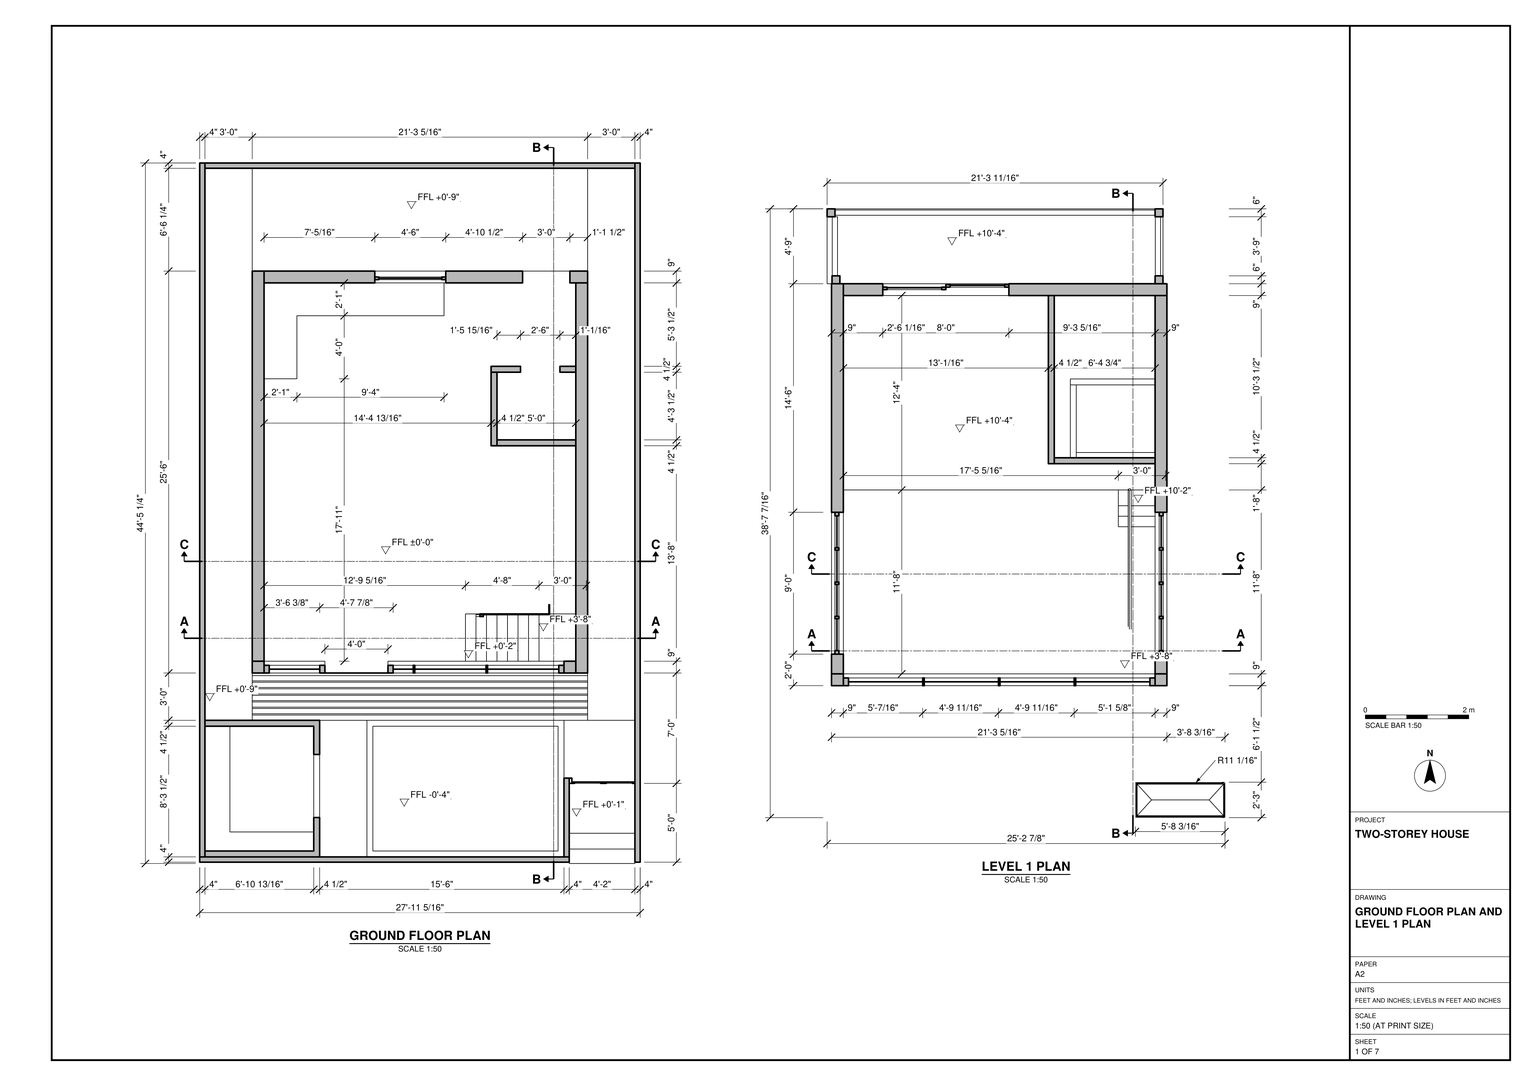
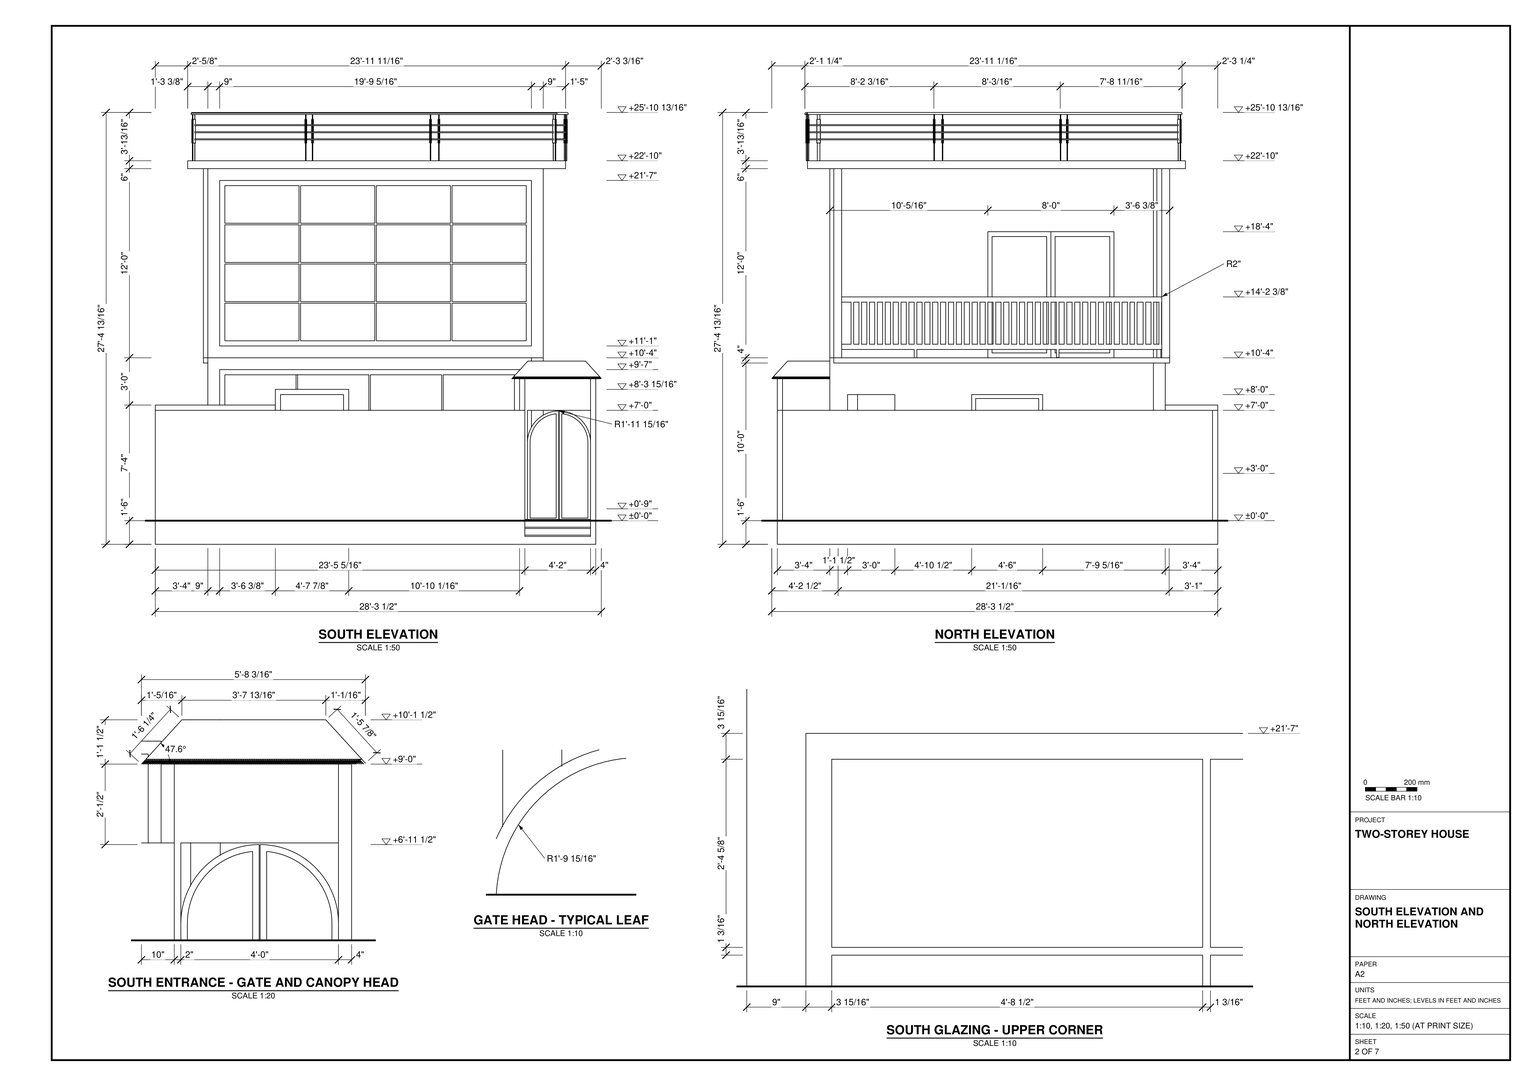
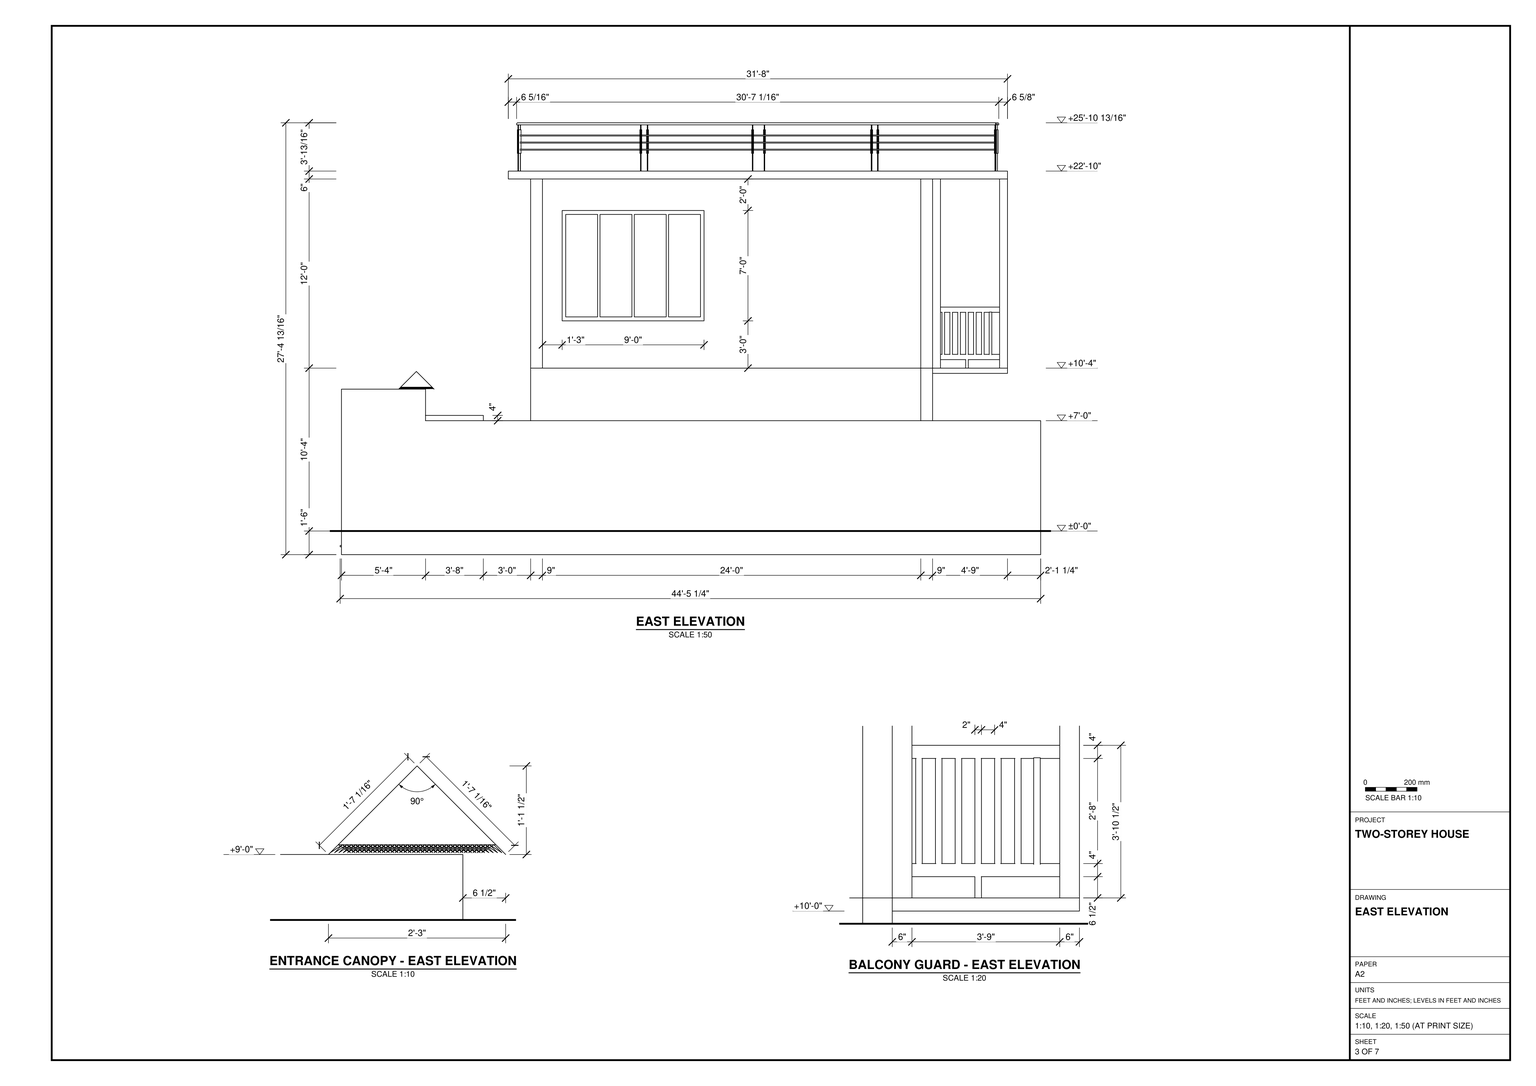
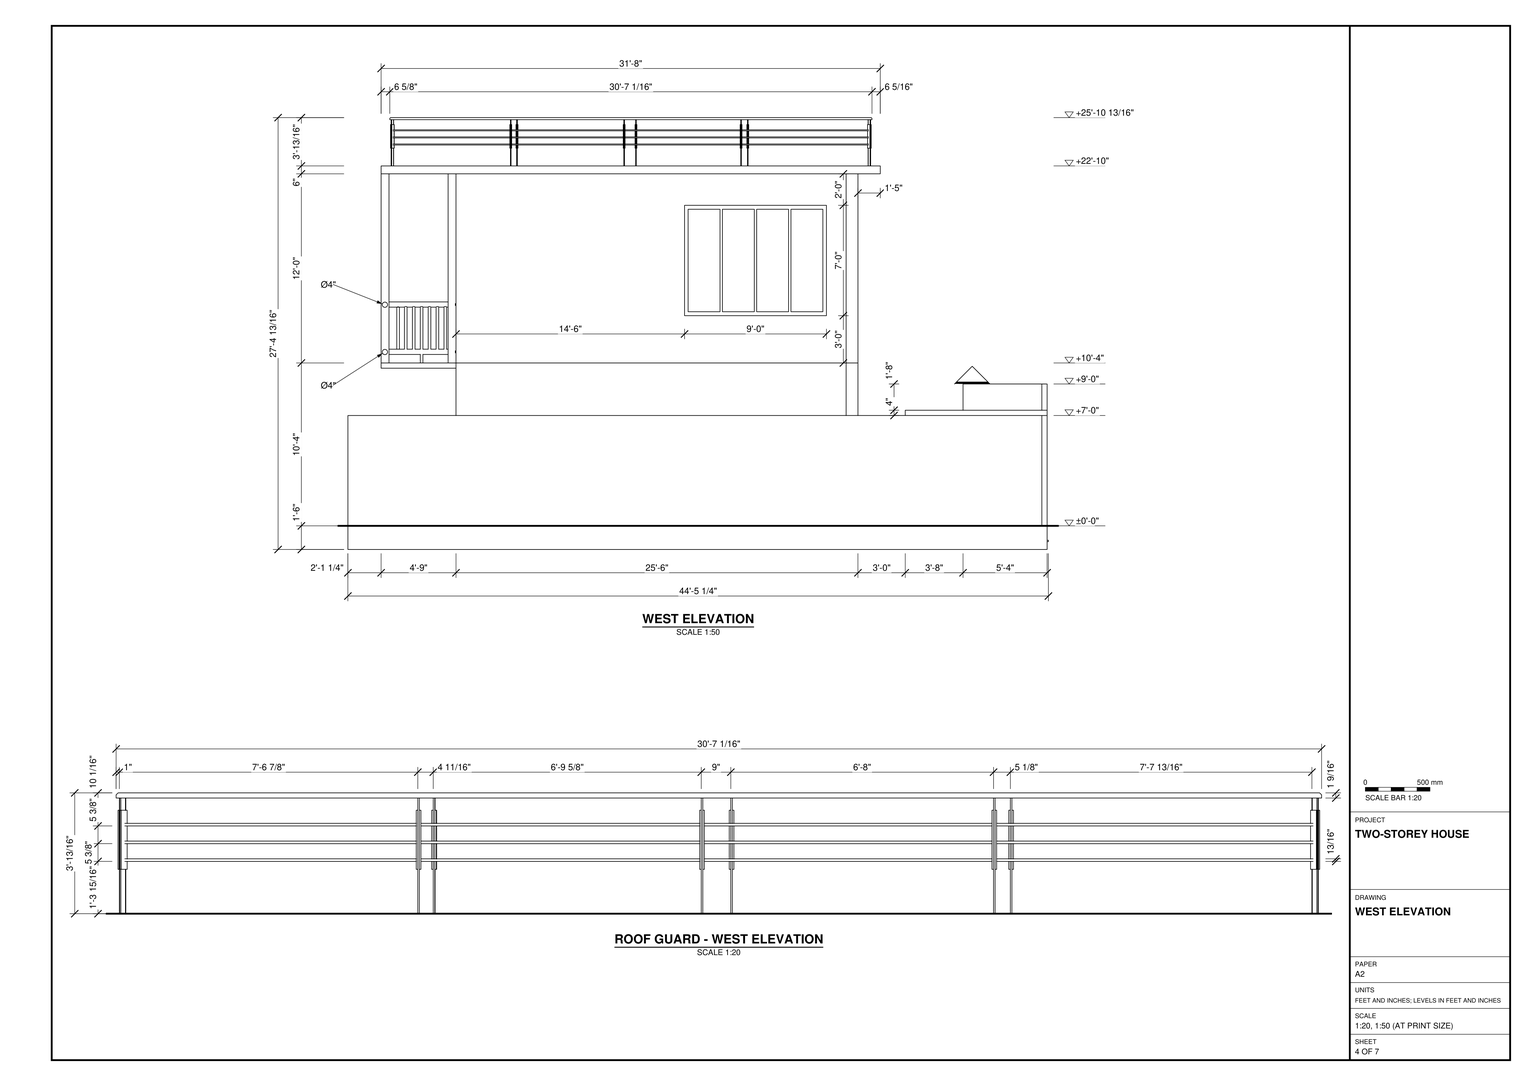
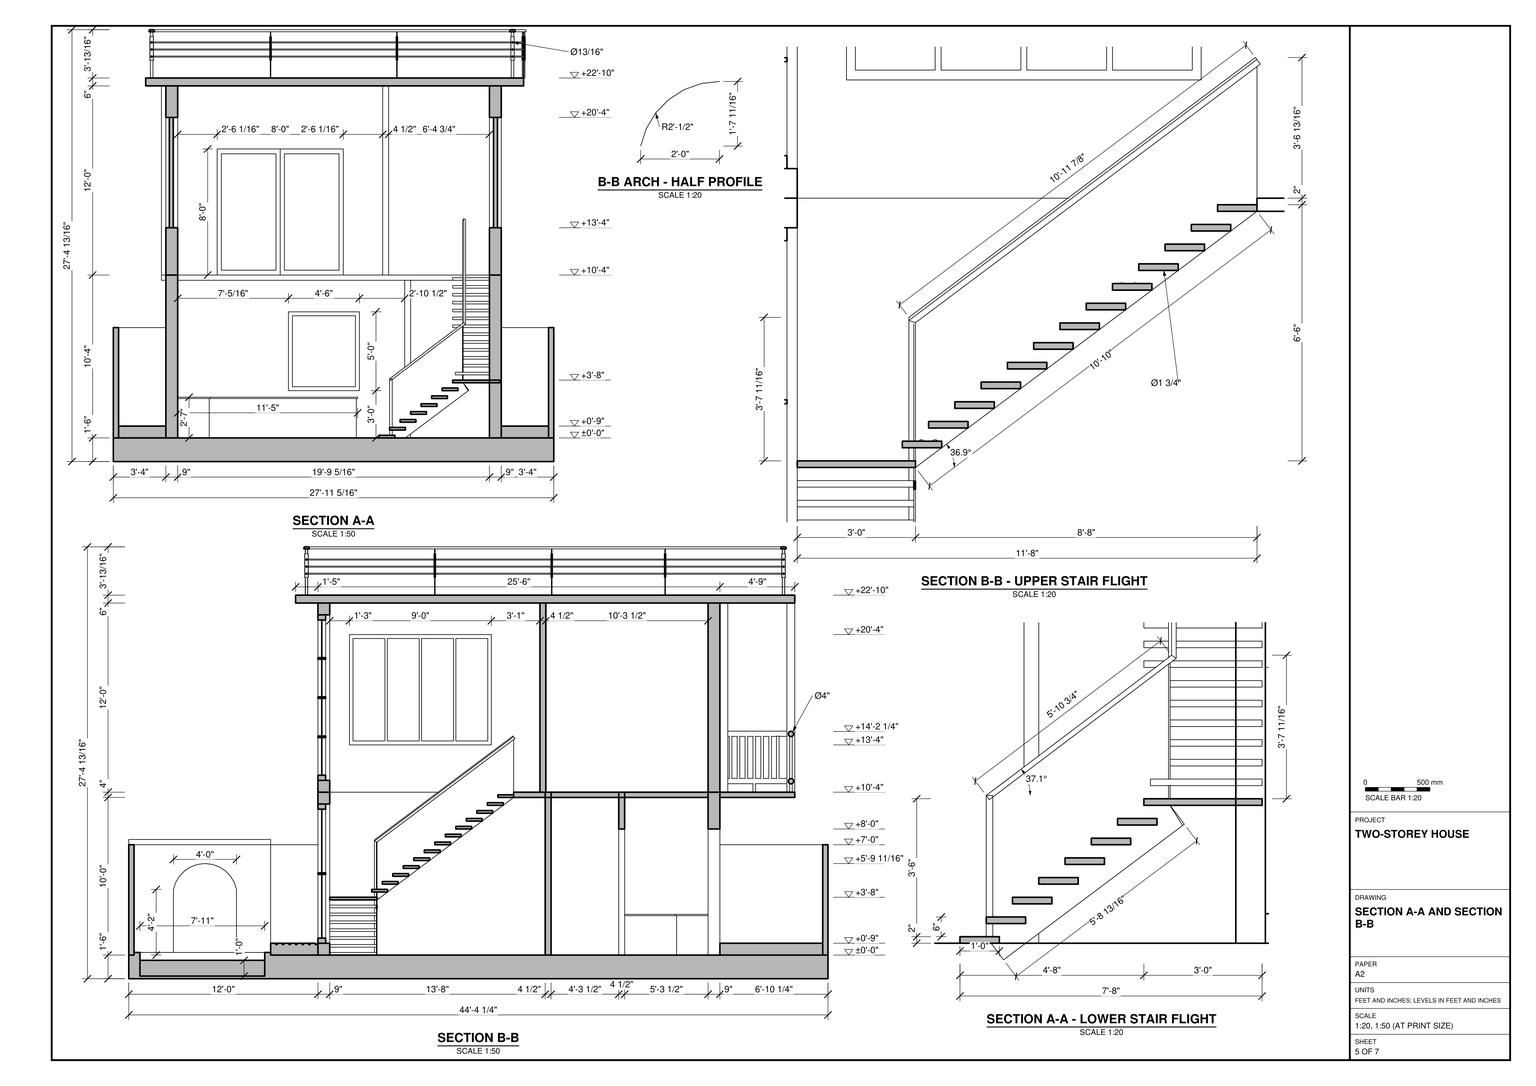
Build the house and its walled court in SketchUp using task_files/diagram_01.pdf. Work in feet and inches. Orient the model with the south frontage along the x-axis and the site depth along the y-axis. The complete model, including the site base and roof guard, is 28'-3 1/2" wide, 44'-5 1/4" deep and 27'-4 13/16" high. Set the ground floor at ±0'-0" and the upper floor at +10'-4".

Lay out the site walls, rectangular pool, adjacent enclosure and stepped approach between the south gate and the house. Give the gate its paired arched leaves and small pitched canopy. Build the floor slabs, exterior walls and interior partitions to the thicknesses drawn. Fit the stair and landings along the east side, leaving the south part of the interior open to the floor below. Match the door and window openings to the plans and elevations, including the grid of glazing on the upper south face. Model the projecting north balcony with its vertical guard members and the flat roof with its horizontal rails. Include built-in joinery and main furniture where shown, following their drawn footprints. Decor and loose items may be any suitable library components.

Keep shell elements and individual furniture or joinery pieces in separate groups or components, and use components for repeated parts. Save one SketchUp model as output_files/two_storey_house_with_a_gated_pool_court.skp.

# SketchUp Ruby script. Lengths in inches.
U = 1.inch
M = Sketchup.active_model
def pt(a) = Geom::Point3d.new(a.map { |v| v * U })
def face(e, loops, mat)
  f = e.add_face(loops[0].map { |a| pt(a) })
  loops[1..].each { |l| e.add_face(l.map { |a| pt(a) }).erase! }
  f.material = f.back_material = mat if mat
  f
end
# faces: each face lists its corners as indices into pts; further lists are holes
def faces(e, pts, list, mat = nil) = list.each { |f| face(e, (f[0].is_a?(Array) ? f : [f]).map { |l| l.map { |i| pts[i] } }, mat) }
# xy, xz, yz: faces in a plane at the given z, y or x. An outline is a flat list of corners, or four numbers for a rectangle; further outlines are holes
def ring(l) = l.size == 4 ? [[l[0], l[1]], [l[2], l[1]], [l[2], l[3]], [l[0], l[3]]] : l.each_slice(2).to_a
def flat(e, list, mat, &to3) = list.each { |f| face(e, (f[0].is_a?(Array) ? f : [f]).map { |l| ring(l).map { |u, v| to3.(u, v) } }, mat) }
def xy(e, z, list, mat = nil) = flat(e, list, mat) { |x, y| [x, y, z] }
def xz(e, y, list, mat = nil) = flat(e, list, mat) { |x, z| [x, y, z] }
def yz(e, x, list, mat = nil) = flat(e, list, mat) { |y, z| [x, y, z] }
def lines(e, pts, list) = list.each { |a, b| e.add_line(pt(pts[a]), pt(pts[b])) }
# prism: a flat outline (further loops are holes) pulled along v
def prism(e, loops, v, mat = nil)
  f = face(e, loops, mat); d = Geom::Vector3d.new(v.map { |x| x * U })
  f.pushpull(f.normal.samedirection?(d) ? d.length : -d.length)
end
def box(e, o, s, mat = nil) = prism(e, [[o, [o[0] + s[0], o[1], o[2]], [o[0] + s[0], o[1] + s[1], o[2]], [o[0], o[1] + s[1], o[2]]]], [0, 0, s[2]], mat)
def at(x, y, z, deg = 0) = Geom::Transformation.translation(pt([x, y, z])) * Geom::Transformation.rotation(ORIGIN, Z_AXIS, deg.degrees)
def axes(o, x, y, z) = Geom::Transformation.new([*x, 0, *y, 0, *z, 0, *pt(o).to_a, 1])
def part(name) = M.definitions.add(name)
# library, detail: a bought-in or finely detailed component or shape, given as its bounding box
def library(name, o, s) = part(name).tap { |d| box(d.entities, o, s) }
def detail(e, o, s) = box(e.add_group.entities, o, s)
def put(e, d, t, mat = nil) = e.add_instance(d, t).tap { |i| i.material = mat if mat }
def group(e, t, mat = nil) = e.add_group.tap { |g| g.transformation = t; g.material = mat if mat }.entities
root = M.entities
M.materials.add("  cane").color = [150, 130, 69]
M.materials.add("[Aluminum]").color = [179, 179, 179]
M.materials.add("[Color A01]").color = [255, 204, 204]
M.materials.add("[Color A08]").color = [102, 0, 0]
M.materials.add("[Color C07]").color = [153, 76, 0]
M.materials.add("[Color F02]").color = [204, 255, 153]
M.materials.add("[Color M02]").color = [198, 198, 198]
M.materials.add("[Color M04]").color = [142, 142, 142]
M.materials.add("[Color M06]").color = [86, 86, 86]
M.materials.add("[Color M07]").color = [58, 58, 58]
M.materials.add("[Color M08]").color = [30, 30, 30]
M.materials.add("[Translucent Glass Gray]").color = [128, 128, 128]
M.materials["[Translucent Glass Gray]"].alpha = 0.1
M.materials.add("[Translucent Glass Gray]1").color = [128, 128, 128]
M.materials["[Translucent Glass Gray]1"].alpha = 0.5
M.materials.add("[Water Pool]").color = [64, 149, 167]
M.materials.add("[Wood Veneer 01]").color = [120, 70, 37]
M.materials.add("[Wood Veneer 02]").color = [190, 128, 91]
c1 = part("Group60\#2")
xy(c1.entities,0,[[-110.22,-49.0625,-71.78,-0.59],[-15.9,-49.0625,-0.59,-0.59],[0.59,-49.0625,54.8125,-0.59],[56,-49.0625,110.22,-0.59],[-110.22,-0.59,-71.78,0.59],
  [-110.22,0.59,-110.22,49.0625,-56,49.0625,-56,37.9375,-71.78,37.9375,-71.78,0.59],[-15.9,0.59,-15.9,37.9375,-54.8125,37.9375,-54.8125,49.0625,-0.59,49.0625,-0.59,0.59],[0.59,0.59,54.8125,49.0625],[56,0.59,110.22,49.0625],[-56,37.9375,-54.8125,49.0625]])
c2 = part("Group59\#1")
xy(c2.entities,0,[[[-114.16,-53,-114.16,53,114.16,53,114.16,-53,-19.84,-53,-19.84,34,-67.84,34,-67.84,-53],[-110.22,-49.0625,-71.78,-49.0625,-71.78,37.9375,-15.9,37.9375,-15.9,0.59,-0.59,0.59,-0.59,49.0625,-110.22,49.0625],[56,-49.0625,110.22,-0.59],[0.59,-49.0625,54.8125,-0.59],[56,0.59,110.22,49.0625],[0.59,0.59,54.8125,49.0625],[-15.9,-49.0625,-0.59,-0.59]]])
xy(c2.entities,5.875,[[[-114.16,-53,-67.84,-53,-67.84,34,-19.84,34,-19.84,-53,114.16,-53,114.16,53,-114.16,53],[-110.22,-49.0625,-110.22,49.0625,-0.59,49.0625,-0.59,0.59,-15.9,0.59,-15.9,37.9375,-71.78,37.9375,-71.78,-49.0625],[56,-49.0625,110.22,-0.59],[0.59,-49.0625,54.8125,-0.59],[56,0.59,110.22,49.0625],[0.59,0.59,54.8125,49.0625],[-15.9,-49.0625,-0.59,-0.59]]])
xz(c2.entities,-53,[[-114.16,0,-67.84,5.875],[-19.84,0,114.16,5.875]])
xz(c2.entities,-49.0625,[[-110.22,0,-71.78,5.875],[-15.9,0,-0.59,5.875],[0.59,0,54.8125,5.875],[56,0,110.22,5.875]])
xz(c2.entities,-0.59,[[-15.9,0,-0.59,5.875],[0.59,0,54.8125,5.875],[56,0,110.22,5.875]])
xz(c2.entities,0.59,[[-15.9,0,-0.59,5.875],[0.59,0,54.8125,5.875],[56,0,110.22,5.875]])
xz(c2.entities,34,[[-67.84,0,-19.84,5.875]])
xz(c2.entities,37.9375,[[-71.78,0,-15.9,5.875]])
xz(c2.entities,49.0625,[[-110.22,0,-0.59,5.875],[0.59,0,54.8125,5.875],[56,0,110.22,5.875]])
xz(c2.entities,53,[[-114.16,0,114.16,5.875]])
yz(c2.entities,-114.16,[[-53,0,53,5.875]])
yz(c2.entities,-110.22,[[-49.0625,0,49.0625,5.875]])
yz(c2.entities,-71.78,[[-49.0625,0,37.9375,5.875]])
yz(c2.entities,-67.84,[[-53,0,34,5.875]])
yz(c2.entities,-19.84,[[-53,0,34,5.875]])
yz(c2.entities,-15.9,[[-49.0625,0,-0.59,5.875],[0.59,0,37.9375,5.875]])
yz(c2.entities,-0.59,[[-49.0625,0,-0.59,5.875],[0.59,0,49.0625,5.875]])
yz(c2.entities,0.59,[[-49.0625,0,-0.59,5.875],[0.59,0,49.0625,5.875]])
yz(c2.entities,54.8125,[[-49.0625,0,-0.59,5.875],[0.59,0,49.0625,5.875]])
yz(c2.entities,56,[[-49.0625,0,-0.59,5.875],[0.59,0,49.0625,5.875]])
yz(c2.entities,110.22,[[-49.0625,0,-0.59,5.875],[0.59,0,49.0625,5.875]])
yz(c2.entities,114.16,[[-53,0,53,5.875]])
put(c2.entities,c1,at(0,0,2.9375),"[Translucent Glass Gray]1")
c3 = part("Group\#217")
detail(c3.entities,[0,0,0],[0.25,1.75,1.75])
c4 = part("Group\#219")
put(c4.entities,c3,at(0,1.625,0))
put(c4.entities,c3,at(0,5.8125,0))
c5 = part("Group\#83")
box(c5.entities,[0,4,0],[45,12,2])
c6 = part("Group\#196")
box(c6.entities,[0,4,0],[45,12,2])
c7 = part("Group44\#2")
xy(c7.entities,0,[[-114.72,-59.0625,-58.25,-30.42],[-57.0625,-59.0625,-0.59,-30.42],[0.59,-59.0625,57.0625,-30.42],[58.25,-59.0625,114.72,-30.42],[-114.72,-29.23,-58.25,-0.59],
  [-57.0625,-29.23,-0.59,-0.59],[0.59,-29.23,57.0625,-0.59],[58.25,-29.23,114.72,-0.59],[-114.72,0.59,-58.25,29.23],[-57.0625,0.59,-0.59,29.23],
  [0.59,0.59,57.0625,29.23],[58.25,0.59,114.72,29.23],[-114.72,30.42,-58.25,59.0625],[-57.0625,30.42,-0.59,59.0625],[0.59,30.42,57.0625,59.0625],
  [58.25,30.42,114.72,59.0625]])
c8 = part("Group43\#1")
prism(c8.entities,[[[118.66,63,0],[118.66,-63,0],[-118.66,-63,0],[-118.66,63,0]],[[-58.25,29.23,0],[-114.72,29.23,0],[-114.72,0.59,0],[-58.25,0.59,0]],[[114.72,-30.42,0],[58.25,-30.42,0],[58.25,-59.0625,0],[114.72,-59.0625,0]],[[58.25,-29.23,0],[114.72,-29.23,0],[114.72,-0.59,0],[58.25,-0.59,0]],[[-114.72,-29.23,0],[-58.25,-29.23,0],[-58.25,-0.59,0],[-114.72,-0.59,0]],[[58.25,0.59,0],[114.72,0.59,0],[114.72,29.23,0],[58.25,29.23,0]],[[57.0625,29.23,0],[0.59,29.23,0],[0.59,0.59,0],[57.0625,0.59,0]],[[-57.0625,29.23,0],[-57.0625,0.59,0],[-0.59,0.59,0],[-0.59,29.23,0]],[[-57.0625,-30.42,0],[-57.0625,-59.0625,0],[-0.59,-59.0625,0],[-0.59,-30.42,0]],[[0.59,30.42,0],[57.0625,30.42,0],[57.0625,59.0625,0],[0.59,59.0625,0]],[[-58.25,30.42,0],[-58.25,59.0625,0],[-114.72,59.0625,0],[-114.72,30.42,0]],[[0.59,-29.23,0],[57.0625,-29.23,0],[57.0625,-0.59,0],[0.59,-0.59,0]],[[-57.0625,-29.23,0],[-0.59,-29.23,0],[-0.59,-0.59,0],[-57.0625,-0.59,0]],[[114.72,30.42,0],[114.72,59.0625,0],[58.25,59.0625,0],[58.25,30.42,0]],[[-114.72,-30.42,0],[-114.72,-59.0625,0],[-58.25,-59.0625,0],[-58.25,-30.42,0]],[[-0.59,30.42,0],[-0.59,59.0625,0],[-57.0625,59.0625,0],[-57.0625,30.42,0]],[[57.0625,-59.0625,0],[57.0625,-30.42,0],[0.59,-30.42,0],[0.59,-59.0625,0]]],[0,0,5.875])
put(c8.entities,c7,at(0,0,2.9375),"[Translucent Glass Gray]1")
c9 = library("Group\#54",[0,0,0],[48,1,83.5])
c10 = part("Group169\#2")
xy(c10.entities,0,[[-57,-39,-30,39],[-28,-39,-1,39],[1,-39,28,39],[30,-39,57,39]])
c11 = part("Group168\#2")
prism(c11.entities,[[[60,-42,0],[-60,-42,0],[-60,42,0],[60,42,0]],[[1,-39,0],[28,-39,0],[28,39,0],[1,39,0]],[[-28,-39,0],[-1,-39,0],[-1,39,0],[-28,39,0]],[[30,39,0],[30,-39,0],[57,-39,0],[57,39,0]],[[-30,-39,0],[-30,39,0],[-57,39,0],[-57,-39,0]]],[0,0,3])
put(c11.entities,c10,at(0,0,1.5),"[Translucent Glass Gray]")
c12 = part("Group1075\#2")
xy(c12.entities,0,[[-19.5,-36,19.5,36]])
c13 = part("Group1074\#1")
prism(c13.entities,[[[22.5,-39,1],[-22.5,-39,1],[-22.5,39,1],[22.5,39,1]],[[-19.5,-36,1],[19.5,-36,1],[19.5,36,1],[-19.5,36,1]]],[0,0,1.9])
put(c13.entities,c12,at(0,0,1.5),"  cane")
c14 = library("Group\#35",[-11.82,0,0],[51,6,144])
c15 = part("Round baluster")
detail(c15.entities,[0,0,0],[2,2,34.375])
c16 = library("Group\#36",[-11.82,0,0],[51,6,144])
c17 = library("Group\#345",[0,0,0],[93.38,26.98,13.49])
c18 = part("Group\#43")
box(c18.entities,[0,0,0],[36,420.27,9])
c19 = library("Group\#46",[0,0,0],[287.05,367.0625,20.87])
c20 = part("Ploe")
box(c20.entities,[613.49,497.4375,274],[0.47,1.97,36])
box(c20.entities,[613.02,497.16,287.5],[0.47,2.52,18],"[Wood Veneer 02]")
box(c20.entities,[613.96,497.16,287.5],[0.48,2.52,18],"[Wood Veneer 02]")
c21 = part("Group91\#1")
put(c21.entities,c20,at(0,0,0))
put(c21.entities,c20,at(1131.02,996.85,0,-180))
put(c21.entities,c20,at(-192.625,0,0))
put(c21.entities,c20,at(249.07,-287.99,0,45))
put(c21.entities,c20,at(829.03,-205.43,0,90))
put(c21.entities,c20,at(-167.82,935.71,0,-90))
put(c21.entities,c20,at(829.03,-380.74,0,90))
put(c21.entities,c20,at(1117.01,53.77,0,135))
put(c21.entities,c20,at(1029.71,633.72,0,180))
put(c21.entities,c20,at(-102.8125,-363.125,0))
put(c21.entities,c20,at(523.76,-651.11,0,45))
put(c21.entities,c20,at(1103.71,-385.87,0,90))
put(c21.entities,c20,at(106.87,926.71,0,-90))
put(c21.entities,c20,at(1075.91,-231.75,0,87.45))
put(c21.entities,c20,at(171.84,1153.6875,0,-95.101))
c22 = part("Group96\#1")
p = [[-3,57,0],[-3,3,0],[-51,3,0],[-51,57,0]]
lines(c22.entities,p,[[0,1],[1,2],[2,3],[3,0]])
c23 = part("Group97\#1")
xy(c23.entities,1,[[-51,3,-3,57]])
c24 = part("Group95\#1")
prism(c24.entities,[[[-54,60,0],[0,60,0],[0,0,0],[-54,0,0]],[[-3,57,0],[-51,57,0],[-51,3,0],[-3,3,0]]],[0,0,2])
put(c24.entities,c22,at(0,0,0))
put(c24.entities,c23,at(0,0,0),"[Translucent Glass Gray]")
xz(root,145,[[95.32,8,143.32,96]],"[Translucent Glass Gray]1")
p = [[187.32,451,96],[187.32,451,36],[133.32,451,36],[133.32,451,96]]
lines(root,p,[[0,1],[1,2],[2,3],[3,0]])
g1 = group(root,at(40,145,0),"[Color M02]")
prism(g1,[[[55.32,0,0],[55.32,0,9],[9,0,9],[9,0,115],[237.32,0,115],[237.32,0,9],[103.32,0,9],[103.32,0,0],[246.32,0,0],[246.32,0,124],[0,0,124],[0,0,0]]],[0,9,0])
put(g1,c2,axes([123.16,5.875,62],[1,0,0],[0,0,1],[0,-1,0]),"[Color M06]")
g2 = group(root,at(40,145,0),"[Color M02]")
xy(g2,0,[[246.32,0,255.32,297],[0,9,9,306],[9,297,205.82,306],[241.82,297,255.32,306]])
xy(g2,36,[[93.32,297,147.32,306]])
xy(g2,96,[[93.32,297,147.32,306],[205.82,297,241.82,306]])
xy(g2,124,[[246.32,0,255.32,297],[0,9,9,306],[9,297,255.32,306]])
xz(g2,0,[[246.32,0,255.32,124]])
xz(g2,9,[[0,0,9,124]])
xz(g2,297,[[[9,0,205.82,0,205.82,96,241.82,96,241.82,0,246.32,0,246.32,124,9,124],[93.32,36,147.32,96]],[246.32,0,255.32,124]])
xz(g2,306,[[0,0,9,124],[[9,0,9,124,255.32,124,255.32,0,241.82,0,241.82,96,205.82,96,205.82,0],[93.32,36,147.32,96]]])
yz(g2,0,[[9,0,306,124]])
yz(g2,9,[[9,0,297,124],[297,0,306,124]])
yz(g2,93.32,[[297,36,306,96]])
yz(g2,147.32,[[297,36,306,96]])
yz(g2,205.82,[[297,0,306,96]])
yz(g2,241.82,[[297,0,306,96]])
yz(g2,246.32,[[0,0,297,124]])
yz(g2,255.32,[[0,0,297,124],[297,0,306,124]])
g3 = group(root,at(221.82,273.5,0),"[Color M02]")
box(g3,[0,44.5,0],[4.5,56,124])
g4 = group(root,at(221.82,374,0),"[Color M02]")
prism(g4,[[[64.5,4.5,0],[52.41,4.5,0],[52.41,4.5,96],[22.41,4.5,96],[22.41,4.5,0],[0,4.5,0],[0,4.5,124],[64.5,4.5,124]]],[0,-4.5,0])
g5 = group(root,at(226.32,318,0),"[Color M02]")
box(g5,[0,0,0],[60,4.5,124])
g6 = group(root,at(210.32,188,2),"[Wood Veneer 01]")
xy(g6,0,[[0,0,2,2]])
xy(g6,43,[[0,0,2,2]])
xz(g6,0,[[0,0,2,0,2,42.51,0.96,41.73,0,43],[0.96,41.73,2,42.51,2,43,0,43],[2,42.51,57.85,84.78,56.4375,85.71,0,43,2,43]])
xz(g6,2,[[0,0,0,43,0.96,41.73,2,42.51,2,0],[0.96,41.73,0,43,2,43,2,42.51],[2,42.51,2,43,0,43,55.5,85,56.91,84.07]])
yz(g6,0,[[0,0,2,43]])
yz(g6,2,[[0,0,2,43]])
p = [[0.96,0,41.73],[0,0,43],[0,2,43],[0.96,2,41.73],[2,2,42.51],[56.91,2,84.07],
  [57.85,0,84.78],[2,0,42.51],[56.4375,0,85.71],[55.5,2,85],[56.91,107.01,162.82],[57.85,105.95,164.24],
  [55.5,106.5625,163.42],[56.4375,105.5,164.84]]
faces(g6,p,[[0,1,2,3],[0,3,4,5,6,7],[2,1,8,9],[6,5,10,11],[5,9,12,10],[8,6,11,13],[9,8,13,12],[13,11,10,12]])
g7 = group(root,at(265.72,190.92,48.72),"[Color M02]")
put(g7,c4,at(0,4.4375,5.55),"[Aluminum]")
put(g7,c4,at(0,12.37,11.55),"[Aluminum]")
put(g7,c4,at(0.09,-1.625,0),"[Aluminum]")
put(g7,c4,at(0,20.42,17.25),"[Aluminum]")
put(g7,c4,at(0,28.03,23.45),"[Aluminum]")
put(g7,c4,at(0,35.96,29.4375),"[Aluminum]")
put(g7,c4,at(0,43.96,35.55),"[Aluminum]")
put(g7,c4,at(0.09,51.41,41.41),"[Aluminum]")
put(g7,c4,at(0.09,59.36,47.78),"[Aluminum]")
put(g7,c4,at(0.09,68.1,53.375),"[Aluminum]")
put(g7,c4,at(0.09,76.51,59.55),"[Aluminum]")
put(g7,c4,at(0.09,92.7,71.5),"[Aluminum]")
put(g7,c4,at(0.09,84.5,65.45),"[Aluminum]")
g8 = group(root,at(189.68,189.5,0.72),"[Translucent Glass Gray]1")
xy(g8,1.28,[[20.64,0,22.14,0.5]],"[Translucent Glass Gray]")
xy(g8,44.28,[[20.64,0,22.14,0.5]],"[Translucent Glass Gray]")
xy(g8,85.9,[[76.14,0,76.64,0.5]],"[Translucent Glass Gray]")
xz(g8,0,[[80.46,35.14,80.96,35.52,76.64,41.28,76.64,41.95,76.14,41.95]])
xz(g8,0,[[25.92,-5.76,80.46,35.14,76.14,41.95,76.14,85.9,20.64,44.28,22.14,44.28,22.14,1.28,20.64,1.28],[76.14,41.95,76.64,85.9]],"[Translucent Glass Gray]")
xz(g8,0.5,[[25.92,-5.76,20.64,1.28,22.14,1.28,22.14,44.28,20.64,44.28,76.14,85.9,76.64,85.9,76.64,41.28,80.96,35.52],[76.14,85.9,76.64,86.28,76.14,86.28],[76.14,85.9,76.64,86.28,76.64,85.9]],"[Translucent Glass Gray]")
xz(g8,104.5,[[76.14,119.28,76.64,123.78],[76.14,123.78,76.64,163.125]],"[Translucent Glass Gray]")
yz(g8,22.14,[[0,1.28,0.5,44.28]],"[Translucent Glass Gray]")
yz(g8,76.14,[[0,85.9,0.5,86.28,0.5,85.9]])
yz(g8,76.14,[[0.5,41.28,0,41.95,0,85.9,0.5,85.9,0.5,86.28,103.95,163.86,104.5,163.125,104.5,119.28]],"[Translucent Glass Gray]")
yz(g8,76.64,[[0,41.28,0.5,41.28,0,41.95],[0,85.9,0.5,85.9,0.5,86.28]])
yz(g8,76.64,[[0.5,41.28,0.5,41.95,0,41.95],[0.5,41.28,104.5,119.28,104.5,163.125,103.95,163.86,0.5,86.28],[0,41.95,0.5,85.9]],"[Translucent Glass Gray]")
p = [[25.92,0,-5.76],[20.64,0,1.28],[20.64,0.5,1.28],[25.92,0.5,-5.76],[80.96,0.5,35.52],[80.96,0,35.52],
  [80.46,0,35.14],[76.64,0.5,41.28],[76.64,0,41.28],[76.14,0.5,41.28],[76.64,0,41.95],[76.14,0,41.95],
  [76.14,104.5,119.28],[76.64,104.5,119.28],[20.64,0,44.28],[76.14,0,85.9],[76.14,0.5,85.9],[20.64,0.5,44.28],
  [76.14,0.5,86.28],[76.64,0,85.9],[76.64,0.5,86.28],[76.64,103.95,163.86],[76.14,103.95,163.86],[76.64,104.5,163.125],
  [76.14,104.5,163.125]]
faces(g8,p,[[0,1,2,3],[9,7,10,11],[9,12,13,7],[14,15,16,17],[21,22,18,20],[23,24,22,21]],"[Translucent Glass Gray]")
faces(g8,p,[[0,3,4,5,6],[7,8,5,4],[18,15,19,20]])
g9 = group(root,at(218.32,154,12),"[Color M02]")
put(g9,c5,axes([76,56,42],[-0.8,0,0],[0,-1,0],[0,0,1]),"[Wood Veneer 01]")
put(g9,c5,axes([40,0,18],[0,0.8,0],[-1,0,0],[0,0,1]),"[Wood Veneer 01]")
put(g9,c5,axes([76,72,54],[-0.8,0,0],[0,-1,0],[0,0,1]),"[Wood Veneer 01]")
put(g9,c5,axes([76,64,48],[-0.8,0,0],[0,-1,0],[0,0,1]),"[Wood Veneer 01]")
put(g9,c5,axes([76,80,60],[-0.8,0,0],[0,-1,0],[0,0,1]),"[Wood Veneer 01]")
put(g9,c5,axes([32,0,12],[0,0.8,0],[-1,0,0],[0,0,1]),"[Wood Veneer 01]")
put(g9,c5,axes([48,0,24],[0,0.8,0],[-1,0,0],[0,0,1]),"[Wood Veneer 01]")
g10 = group(g9,at(76,48,36),"[Wood Veneer 01]")
box(g10,[-34,-16,0],[34,12,2])
put(g9,c6,axes([16,0,0],[0,0.8,0],[-1,0,0],[0,0,1]),"[Wood Veneer 01]")
g11 = group(g9,at(24,0,6),"[Wood Veneer 01]")
box(g11,[-16,0,0],[12,36,2])
put(g9,c5,axes([76,96,72],[-0.8,0,0],[0,-1,0],[0,0,1]),"[Wood Veneer 01]")
put(g9,c5,axes([76,88,66],[-0.8,0,0],[0,-1,0],[0,0,1]),"[Wood Veneer 01]")
put(g9,c5,axes([76,144,108],[-0.8,0,0],[0,-1,0],[0,0,1]),"[Wood Veneer 01]")
put(g9,c5,axes([76,104,78],[-0.8,0,0],[0,-1,0],[0,0,1]),"[Wood Veneer 01]")
put(g9,c5,axes([76,128,96],[-0.8,0,0],[0,-1,0],[0,0,1]),"[Wood Veneer 01]")
put(g9,c5,axes([76,112,84],[-0.8,0,0],[0,-1,0],[0,0,1]),"[Wood Veneer 01]")
put(g9,c5,axes([76,136,102],[-0.8,0,0],[0,-1,0],[0,0,1]),"[Wood Veneer 01]")
put(g9,c5,axes([76,120,90],[-0.8,0,0],[0,-1,0],[0,0,1]),"[Wood Veneer 01]")
g12 = group(g9,at(40,0,30),"[Wood Veneer 01]")
box(g12,[0,0,0],[36,36,2])
put(g9,c6,axes([8,0,-6],[0,0.8,0],[-1,0,0],[0,0,1]),"[Wood Veneer 01]")
put(g9,c6,axes([0,0,-12],[0,0.8,0],[-1,0,0],[0,0,1]),"[Wood Veneer 01]")
g13 = group(root,at(49,278,120),"[Color M02]")
box(g13,[0,16,0],[237.32,148,4])
g14 = group(root,at(40,145,124),"[Color M02]")
g15 = group(g14,at(0,255.32,0,-90))
prism(g15,[[[246.32,9,0],[-50.68,9,0],[-50.68,9,144],[246.32,9,144]],[[123.32,9,120],[123.32,9,36],[231.32,9,36],[231.32,9,120]]],[0,-9,0])
g16 = group(g14,at(246.32,9,0))
prism(g16,[[[0,288,0],[0,0,0],[0,0,144],[0,288,144]],[[0,15,36],[0,123,36],[0,123,120],[0,15,120]]],[9,0,0])
g17 = group(g14,at(9,297,0))
prism(g17,[[[0,0,0],[30.03,0,0],[30.03,0,96],[126.03,0,96],[126.03,0,0],[246.32,0,0],[246.32,0,144],[0,0,144]]],[0,9,0])
g18 = group(g14,at(-312.1875,0,0))
prism(g18,[[[312.1875,0,0],[567.5,0,0],[567.5,0,144],[312.1875,0,144]],[[558.5,0,9],[321.1875,0,9],[321.1875,0,135],[558.5,0,135]]],[0,9,0])
put(g18,c8,axes([439.85,5.875,72],[1,0,0],[0,0,1],[0,-1,0]),"[Color M07]")
g19 = group(root,at(205.07,314,124),"[Color M02]")
box(g19,[0,0,0],[4.5,128,144])
g20 = group(root,at(209.57,314,124),"[Color M02]")
box(g20,[0,0,0],[76.75,4.5,144])
g21 = group(root,at(40,451,120),"[Color M02]")
box(g21,[-3.37,0,0],[255.69,57,4])
g22 = group(root,at(0,5,0),"[Color M04]")
box(g22,[0,0,0],[4,528.27,84])
g23 = group(root,at(0,1,0),"[Color M04]")
box(g23,[0,0,0],[281.32,4,84])
g24 = group(root,at(331.32,1,0),"[Color M04]")
prism(g24,[[[4,0,0],[4,532.27,0],[4,532.27,84],[4,64,84],[4,64,108],[4,0,108]]],[-4,0,0])
g25 = group(root,at(4,529.27,0),"[Color M04]")
box(g25,[0,0,0],[327.32,4,84])
g26 = group(root,at(0,1,-18),"[Color M04]")
xy(g26,0,[[0,0,335.32,532.27]])
xy(g26,2,[[131.82,8.5,272.82,103.5]])
xy(g26,6,[[281.32,0,331.32,12],[4,8.5,86.82,103.5]])
xy(g26,12,[[281.32,12,331.32,24]])
xy(g26,14,[[131.82,8.5,272.82,103.5]],"[Water Pool]")
xy(g26,18,[[[0,0,281.32,0,281.32,24,331.32,24,331.32,0,335.32,0,335.32,532.27,0,532.27],[127.32,4,277.32,108],[4,8.5,86.82,103.5]]])
xy(g26,20,[[[127.32,4,277.32,108],[131.82,8.5,272.82,103.5]]],"[Color M06]")
xz(g26,0,[[0,0,335.32,0,335.32,18,331.32,18,331.32,6,281.32,6,281.32,18,0,18]],"[Color F02]")
xz(g26,4,[[127.32,18,277.32,20]],"[Color M06]")
xz(g26,8.5,[[131.82,2,272.82,14],[4,6,86.82,18]])
xz(g26,8.5,[[131.82,14,272.82,20]],"[Color M06]")
xz(g26,12,[[281.32,6,331.32,12]],"[Color F02]")
xz(g26,24,[[281.32,12,331.32,18]],"[Color F02]")
xz(g26,103.5,[[131.82,2,272.82,14],[4,6,86.82,18]])
xz(g26,103.5,[[131.82,14,272.82,20]],"[Color M06]")
xz(g26,108,[[127.32,18,277.32,20]],"[Color M06]")
xz(g26,532.27,[[0,0,335.32,18]])
yz(g26,0,[[0,0,532.27,18]])
yz(g26,4,[[8.5,6,103.5,18]])
yz(g26,86.82,[[8.5,6,103.5,18]])
yz(g26,127.32,[[4,18,108,20]],"[Color M06]")
yz(g26,131.82,[[8.5,2,103.5,14],[8.5,14,103.5,20]])
yz(g26,272.82,[[8.5,2,103.5,14]])
yz(g26,272.82,[[8.5,14,103.5,20]],"[Color M06]")
yz(g26,277.32,[[4,18,108,20]],"[Color M06]")
yz(g26,281.32,[[0,6,12,18],[12,12,24,18]])
yz(g26,331.32,[[0,6,12,18],[12,12,24,18]])
yz(g26,335.32,[[0,0,532.27,18]])
g27 = group(root,at(277.32,5,0),"[Color M04]")
box(g27,[0,0,0],[4,60,108])
g28 = group(root,at(281.32,61,0),"[Color M04]")
prism(g28,[[[0,0,0],[2,0,0],[2,0,84],[50,0,84],[50,0,108],[0,0,108]]],[0,4,0])
g29 = group(root,at(281.32,0,-12),"[Color M02]")
box(g29,[0,0,0],[50,13,1])
g30 = group(root,at(281.32,12,-6),"[Color M02]")
box(g30,[0,-1,0],[50,14,1])
g31 = group(root,at(281.32,24,0),"[Color M02]")
box(g31,[0,-1,0],[50,38,1])
put(root,c9,at(283.32,61,0),"[Color M02]")
g32 = group(root,at(91.32,5,0),"[Color M04]")
box(g32,[0,0,0],[36,104,2])
g33 = group(root,at(4,5,0),"[Color M04]")
xy(g33,0,[[0,0,0,4.5,82.82,4.5,82.82,30,87.32,30,87.32,0],[82.82,78,82.82,99.5,0,99.5,0,104,87.32,104,87.32,78]])
xy(g33,84,[[0,0,87.32,0,87.32,104,0,104,0,99.5,82.82,99.5,82.82,4.5,0,4.5]])
xz(g33,0,[[0,0,87.32,84]])
xz(g33,4.5,[[0,0,82.82,84]])
xz(g33,30,[[82.82,0,87.32,50]])
xz(g33,78,[[82.82,0,87.32,50]])
xz(g33,99.5,[[0,0,82.82,84]])
xz(g33,104,[[0,0,87.32,84]])
yz(g33,0,[[0,0,4.5,84],[4.5,0,99.5,84],[99.5,0,104,84]])
yz(g33,82.82,[[4.5,0,4.5,84,99.5,84,99.5,0,78,0,78,50,76.29,55.32,73.41,60.12,69.52,64.14,64.82,67.17,59.56,69.05,54,69.6875,48.44,69.05,43.18,67.17,38.48,64.14,34.59,60.12,31.71,55.32,30,50,30,0]])
yz(g33,87.32,[[0,0,30,0,30,50,31.71,55.32,34.59,60.12,38.48,64.14,43.18,67.17,48.44,69.05,54,69.6875,59.56,69.05,64.82,67.17,69.52,64.14,73.41,60.12,76.29,55.32,78,50,78,0,104,0,104,84,0,84]])
p = [[87.32,31.71,55.32],[87.32,30,50],[82.82,30,50],[82.82,31.71,55.32],[87.32,78,50],[87.32,76.29,55.32],
  [82.82,76.29,55.32],[82.82,78,50],[87.32,34.59,60.12],[82.82,34.59,60.12],[87.32,73.41,60.12],[82.82,73.41,60.12],
  [87.32,38.48,64.14],[82.82,38.48,64.14],[87.32,69.52,64.14],[82.82,69.52,64.14],[87.32,43.18,67.17],[82.82,43.18,67.17],
  [87.32,64.82,67.17],[82.82,64.82,67.17],[87.32,48.44,69.05],[82.82,48.44,69.05],[87.32,59.56,69.05],[82.82,59.56,69.05],
  [87.32,54,69.6875],[82.82,54,69.6875]]
faces(g33,p,[[0,1,2,3],[4,5,6,7],[8,0,3,9],[5,10,11,6],[12,8,9,13],[10,14,15,11],[16,12,13,17],[14,18,19,15],
  [20,16,17,21],[18,22,23,19],[24,20,21,25],[22,24,25,23]])
g34 = group(root,at(40,145,268),"[Color M02]")
box(g34,[-15.37,-17,0],[287.69,380,6])
put(root,c11,axes([45.625,223,202],[0,-0.9,0],[0,0,1],[-1,0,0]),"[Color M07]")
g35 = group(root,at(79.03,446.5,124),"[Color M02]")
put(g35,c13,axes([24,2.9,48],[1.06667,0,0],[0,0,1.23077],[0,-1,0]),"[Color M08]")
put(g35,c13,axes([72,4.8,48],[1.06667,0,0],[0,0,1.23077],[0,-1,0]),"[Color M08]")
put(root,c14,at(286.32,490.18,124,-90),"[Color M02]")
g36 = group(root,at(-42.81,502,124),"[Color M02]")
g37 = group(g36,at(329.125,0,0),"[Color C07]")
box(g37,[0,0,0],[6,6,144])
g38 = group(g36,at(0,1.12,0))
put(g38,c15,axes([139.69,0.98,8.57],[1.00158,0,0],[0,0.96889,0],[0,0,1]),"[Color C07]")
put(g38,c15,axes([97.625,0.98,8.57],[1.00158,0,0],[0,0.96889,0],[0,0,1]),"[Color C07]")
put(g38,c15,axes([175.75,0.98,8.57],[1.00158,0,0],[0,0.96889,0],[0,0,1]),"[Color C07]")
put(g38,c15,axes([169.74,0.98,8.57],[1.00158,0,0],[0,0.96889,0],[0,0,1]),"[Color C07]")
put(g38,c15,axes([121.66,0.98,8.57],[1.00158,0,0],[0,0.96889,0],[0,0,1]),"[Color C07]")
put(g38,c15,axes([91.62,0.98,8.57],[1.00158,0,0],[0,0.96889,0],[0,0,1]),"[Color C07]")
put(g38,c15,axes([127.67,0.98,8.57],[1.00158,0,0],[0,0.96889,0],[0,0,1]),"[Color C07]")
put(g38,c15,axes([247.86,0.98,8.57],[1.00158,0,0],[0,0.96889,0],[0,0,1]),"[Color C07]")
put(g38,c15,axes([313.97,0.98,8.57],[1.00158,0,0],[0,0.96889,0],[0,0,1]),"[Color C07]")
put(g38,c15,axes([271.9,0.98,0],[1.00158,0,0],[0,0.96889,0],[0,0,1.24939]),"[Color C07]")
put(g38,c15,axes([217.82,0.98,8.57],[1.00158,0,0],[0,0.96889,0],[0,0,1]),"[Color C07]")
put(g38,c15,axes([199.79,0.98,8.57],[1.00158,0,0],[0,0.96889,0],[0,0,1]),"[Color C07]")
put(g38,c15,axes([211.81,0.98,8.57],[1.00158,0,0],[0,0.96889,0],[0,0,1]),"[Color C07]")
put(g38,c15,axes([115.66,0.98,8.57],[1.00158,0,0],[0,0.96889,0],[0,0,1]),"[Color C07]")
put(g38,c15,axes([241.85,0.98,8.57],[1.00158,0,0],[0,0.96889,0],[0,0,1]),"[Color C07]")
put(g38,c15,axes([187.77,0.98,8.57],[1.00158,0,0],[0,0.96889,0],[0,0,1]),"[Color C07]")
put(g38,c15,axes([193.79,0.98,8.57],[1.00158,0,0],[0,0.96889,0],[0,0,1]),"[Color C07]")
put(g38,c15,axes([307.96,0.98,8.57],[1.00158,0,0],[0,0.96889,0],[0,0,1]),"[Color C07]")
put(g38,c15,axes([229.84,0.98,8.57],[1.00158,0,0],[0,0.96889,0],[0,0,1]),"[Color C07]")
put(g38,c15,axes([295.94,0.98,8.57],[1.00158,0,0],[0,0.96889,0],[0,0,1]),"[Color C07]")
put(g38,c15,axes([253.875,0.98,8.57],[1.00158,0,0],[0,0.96889,0],[0,0,1]),"[Color C07]")
put(g38,c15,axes([109.65,0.98,8.57],[1.00158,0,0],[0,0.96889,0],[0,0,1]),"[Color C07]")
put(g38,c15,axes([265.89,0.98,8.57],[1.00158,0,0],[0,0.96889,0],[0,0,1]),"[Color C07]")
put(g38,c15,axes([133.68,0.98,8.57],[1.00158,0,0],[0,0.96889,0],[0,0,1]),"[Color C07]")
put(g38,c15,axes([205.8,0.98,8.57],[1.00158,0,0],[0,0.96889,0],[0,0,1]),"[Color C07]")
put(g38,c15,axes([145.7,0.98,8.57],[1.00158,0,0],[0,0.96889,0],[0,0,1]),"[Color C07]")
put(g38,c15,axes([104.25,0.98,8.57],[1.00158,0,0],[0,0.96889,0],[0,0,1]),"[Color C07]")
put(g38,c15,axes([85.61,0.98,8.57],[1.00158,0,0],[0,0.96889,0],[0,0,1]),"[Color C07]")
put(g38,c15,axes([277.91,0.98,8.57],[1.00158,0,0],[0,0.96889,0],[0,0,1]),"[Color C07]")
put(g38,c15,axes([235.85,0.98,8.57],[1.00158,0,0],[0,0.96889,0],[0,0,1]),"[Color C07]")
put(g38,c15,axes([223.83,0.98,8.57],[1.00158,0,0],[0,0.96889,0],[0,0,1]),"[Color C07]")
put(g38,c15,axes([157.72,0.98,8.57],[1.00158,0,0],[0,0.96889,0],[0,0,1]),"[Color C07]")
put(g38,c15,axes([181.76,0.98,8.57],[1.00158,0,0],[0,0.96889,0],[0,0,1]),"[Color C07]")
put(g38,c15,axes([151.71,0.98,8.57],[1.00158,0,0],[0,0.96889,0],[0,0,1]),"[Color C07]")
put(g38,c15,axes([163.65,0.98,0.22],[1.00158,0,0],[0,0.96889,0],[0,0,1.24309]),"[Color C07]")
put(g38,c15,axes([301.95,0.98,8.57],[1.00158,0,0],[0,0.96889,0],[0,0,1]),"[Color C07]")
put(g38,c15,axes([289.93,0.98,8.57],[1.00158,0,0],[0,0.96889,0],[0,0,1]),"[Color C07]")
put(g38,c15,axes([259.88,0.98,8.57],[1.00158,0,0],[0,0.96889,0],[0,0,1]),"[Color C07]")
put(g38,c15,axes([319.98,0.98,8.57],[1.00158,0,0],[0,0.96889,0],[0,0,1]),"[Color C07]")
put(g38,c15,axes([283.92,0.98,8.57],[1.00158,0,0],[0,0.96889,0],[0,0,1]),"[Color C07]")
g39 = group(g38,at(331.85,4,42.35,-180),"[Color C07]")
prism(g39,[[[252.04,2.42,0.04],[252.04,2.62,0.1],[252.04,2.8125,0.17],[252.04,3,0.27],[252.04,3.18,0.38],[252.04,3.34,0.51],[252.04,3.49,0.66],[252.04,3.62,0.82],[252.04,3.73,1],[252.04,3.83,1.1875],[252.04,3.9,1.38],[252.04,3.96,1.58],[252.04,3.99,1.79],[252.04,4,2],[252.04,3.99,2.21],[252.04,3.96,2.42],[252.04,3.9,2.62],[252.04,3.83,2.8125],[252.04,3.73,3],[252.04,3.62,3.18],[252.04,3.49,3.34],[252.04,3.34,3.49],[252.04,3.18,3.62],[252.04,3,3.73],[252.04,2.8125,3.83],[252.04,2.62,3.9],[252.04,2.42,3.96],[252.04,2.21,3.99],[252.04,2,4],[252.04,1.79,3.99],[252.04,1.58,3.96],[252.04,1.38,3.9],[252.04,1.1875,3.83],[252.04,1,3.73],[252.04,0.82,3.62],[252.04,0.66,3.49],[252.04,0.51,3.34],[252.04,0.38,3.18],[252.04,0.27,3],[252.04,0.17,2.8125],[252.04,0.1,2.62],[252.04,0.04,2.42],[252.04,0.01,2.21],[252.04,0,2],[252.04,0.01,1.79],[252.04,0.04,1.58],[252.04,0.1,1.38],[252.04,0.17,1.1875],[252.04,0.27,1],[252.04,0.38,0.82],[252.04,0.51,0.66],[252.04,0.66,0.51],[252.04,0.82,0.38],[252.04,1,0.27],[252.04,1.1875,0.17],[252.04,1.38,0.1],[252.04,1.58,0.04],[252.04,1.79,0.01],[252.04,2,0],[252.04,2.21,0.01]]],[-252.04,0,0])
g40 = group(g38,at(331.85,4,6.35,-180),"[Color C07]")
prism(g40,[[[0,2.62,0.1],[0,2.42,0.04],[0,2.21,0.01],[0,2,0],[0,1.79,0.01],[0,1.58,0.04],[0,1.38,0.1],[0,1.1875,0.17],[0,1,0.27],[0,0.82,0.38],[0,0.66,0.51],[0,0.51,0.66],[0,0.38,0.82],[0,0.27,1],[0,0.17,1.1875],[0,0.1,1.38],[0,0.04,1.58],[0,0.01,1.79],[0,0,2],[0,0.01,2.21],[0,0.04,2.42],[0,0.1,2.62],[0,0.17,2.8125],[0,0.27,3],[0,0.38,3.18],[0,0.51,3.34],[0,0.66,3.49],[0,0.82,3.62],[0,1,3.73],[0,1.1875,3.83],[0,1.38,3.9],[0,1.58,3.96],[0,1.79,3.99],[0,2,4],[0,2.21,3.99],[0,2.42,3.96],[0,2.62,3.9],[0,2.8125,3.83],[0,3,3.73],[0,3.18,3.62],[0,3.34,3.49],[0,3.49,3.34],[0,3.62,3.18],[0,3.73,3],[0,3.83,2.8125],[0,3.9,2.62],[0,3.96,2.42],[0,3.99,2.21],[0,4,2],[0,3.99,1.79],[0,3.96,1.58],[0,3.9,1.38],[0,3.83,1.1875],[0,3.73,1],[0,3.62,0.82],[0,3.49,0.66],[0,3.34,0.51],[0,3.18,0.38],[0,3,0.27],[0,2.8125,0.17]]],[252.04,0,0])
g41 = group(g36,at(79.4375,0,0),"[Color C07]")
box(g41,[0,0,0],[6,6,144])
put(root,c16,at(40.37,490.18,124,-90),"[Color M02]")
put(root,c11,axes([292.44,223,202],[0,-0.9,0],[0,0,1],[-1,0,0]),"[Color M07]")
g42 = group(root,at(40,109,0),"[Color M04]")
prism(g42,[[[0,36,0],[0,0,0],[0,0,9],[0,4,9],[0,4,8],[0,5,8],[0,5,9],[0,9,9],[0,9,8],[0,10,8],[0,10,9],[0,14,9],[0,14,8],[0,15,8],[0,15,9],[0,19,9],[0,19,8],[0,20,8],[0,20,9],[0,24,9],[0,24,8],[0,25,8],[0,25,9],[0,29,9],[0,29,8],[0,30,8],[0,30,9],[0,34,9],[0,34,8],[0,36,8]]],[255.32,0,0])
g43 = group(root,at(49,370,30),"[Color A08]")
prism(g43,[[[0,72,0],[137,72,0],[137,47,0],[25,47,0],[25,-1,0],[0,-1,0]]],[0,0,1])
g44 = group(root,at(0,1,84),"[Color M04]")
box(g44,[0,0,0],[91.32,108,4])
g45 = group(root,at(4,9.5,0),"[Color M04]")
prism(g45,[[[19,95,0],[19,14.5,0],[82.82,14.5,0],[82.82,0,0],[0,0,0],[0,95,0]]],[0,0,1])
g46 = group(root,at(4,9.5,-12),"[Color M04]")
prism(g46,[[[18,95,0],[18,13.5,0],[82.82,13.5,0],[82.82,0,0],[0,0,0],[0,95,0]]],[0,0,12])
put(root,c17,axes([271.32,44.53,108],[0.7304,0,0],[0,1,0],[0,0,1]),"[Color M02]")
put(root,c18,at(4,109,0),"[Color M02]")
put(root,c18,at(295.32,109,0),"[Color M02]")
g47 = group(root,at(40,451,0),"[Color M02]")
box(g47,[0,0,0],[255.32,78.27,9])
g48 = group(root,at(27.22,134.33,274),"[Color M02]")
put(g48,c19,at(0,0,15.92))
put(g48,c21,at(-328.64,-133.33,-274))
g49 = group(root,at(49,370,0),"[Color A01]")
prism(g49,[[[0,72,0],[136,72,0],[136,48,0],[24,48,0],[24,0,0],[0,0,0]]],[0,0,30],"[Color A01]")
put(root,c24,axes([133.32,444.5,36],[-1,0,0],[0,0,1],[0,1,0]),"[Color M06]")
